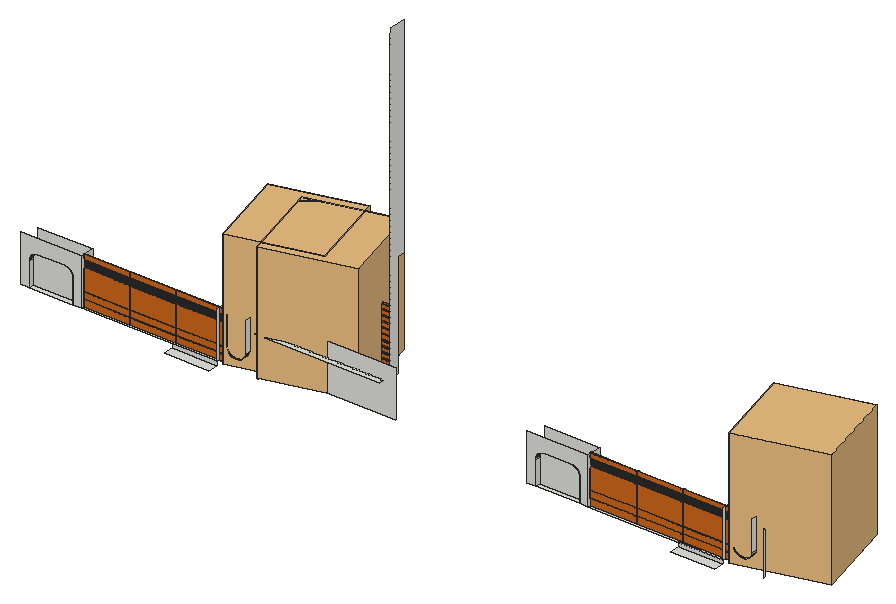
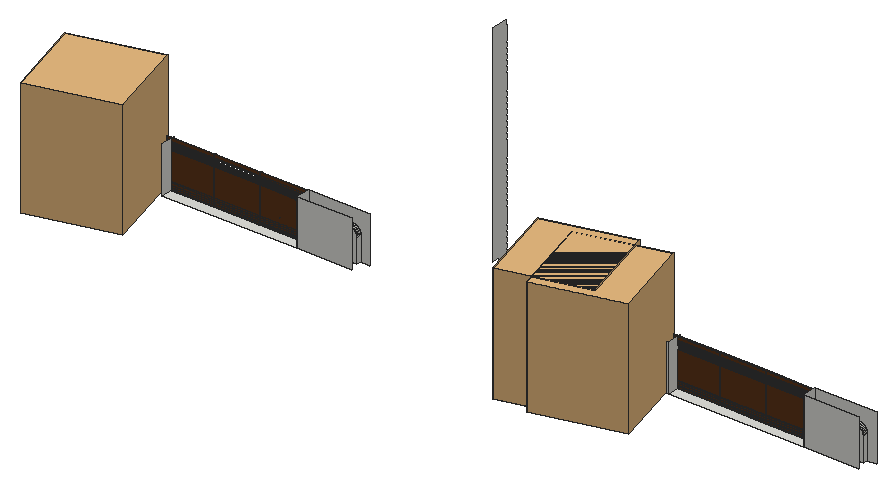
# SketchUp Ruby script. Lengths in inches.
U = 1.inch
M = Sketchup.active_model
def pt(a) = Geom::Point3d.new(a.map { |v| v * U })
def face(e, loops, mat)
  f = e.add_face(loops[0].map { |a| pt(a) })
  loops[1..].each { |l| e.add_face(l.map { |a| pt(a) }).erase! }
  f.material = f.back_material = mat if mat
  f
end
# faces: each face lists its corners as indices into pts; further lists are holes
def faces(e, pts, list, mat = nil) = list.each { |f| face(e, (f[0].is_a?(Array) ? f : [f]).map { |l| l.map { |i| pts[i] } }, mat) }
# xy, xz, yz: faces in a plane at the given z, y or x. An outline is a flat list of corners, or four numbers for a rectangle; further outlines are holes
def ring(l) = l.size == 4 ? [[l[0], l[1]], [l[2], l[1]], [l[2], l[3]], [l[0], l[3]]] : l.each_slice(2).to_a
def flat(e, list, mat, &to3) = list.each { |f| face(e, (f[0].is_a?(Array) ? f : [f]).map { |l| ring(l).map { |u, v| to3.(u, v) } }, mat) }
def xy(e, z, list, mat = nil) = flat(e, list, mat) { |x, y| [x, y, z] }
def xz(e, y, list, mat = nil) = flat(e, list, mat) { |x, z| [x, y, z] }
def yz(e, x, list, mat = nil) = flat(e, list, mat) { |y, z| [x, y, z] }
def lines(e, pts, list) = list.each { |a, b| e.add_line(pt(pts[a]), pt(pts[b])) }
# prism: a flat outline (further loops are holes) pulled along v
def prism(e, loops, v, mat = nil)
  f = face(e, loops, mat); d = Geom::Vector3d.new(v.map { |x| x * U })
  f.pushpull(f.normal.samedirection?(d) ? d.length : -d.length)
end
def box(e, o, s, mat = nil) = prism(e, [[o, [o[0] + s[0], o[1], o[2]], [o[0] + s[0], o[1] + s[1], o[2]], [o[0], o[1] + s[1], o[2]]]], [0, 0, s[2]], mat)
def at(x, y, z, deg = 0) = Geom::Transformation.translation(pt([x, y, z])) * Geom::Transformation.rotation(ORIGIN, Z_AXIS, deg.degrees)
def axes(o, x, y, z) = Geom::Transformation.new([*x, 0, *y, 0, *z, 0, *pt(o).to_a, 1])
def part(name) = M.definitions.add(name)
# library, detail: a bought-in or finely detailed component or shape, given as its bounding box
def library(name, o, s) = part(name).tap { |d| box(d.entities, o, s) }
def detail(e, o, s) = box(e.add_group.entities, o, s)
def put(e, d, t, mat = nil) = e.add_instance(d, t).tap { |i| i.material = mat if mat }
def group(e, t, mat = nil) = e.add_group.tap { |g| g.transformation = t; g.material = mat if mat }.entities
root = M.entities
M.materials.add("[0041_Chocolate]").color = [210, 105, 30]
M.materials.add("[Color M06]").color = [84, 84, 84]
M.materials.add("[Wood Veneer 01]2").color = [94, 55, 29]
c1 = part("Slatted screen panel")
xy(c1.entities,0,[[0,0,255.91,1.97]],"[Wood Veneer 01]2")
xy(c1.entities,16.54,[[0,1.18,255.91,1.97]],"[Wood Veneer 01]2")
xy(c1.entities,16.93,[[0,0,255.91,1.18]],"[Wood Veneer 01]2")
xy(c1.entities,17.78,[[0,0,255.91,1.18]],"[Wood Veneer 01]2")
xy(c1.entities,34.45,[[0,0,255.91,1.18]],"[Wood Veneer 01]2")
xy(c1.entities,35.07,[[0,0,255.91,1.18]],"[Wood Veneer 01]2")
xy(c1.entities,89.37,[[0,0,255.91,1.97]],"[Wood Veneer 01]2")
xy(c1.entities,92.91,[[0,0,255.91,1.97]],"[Wood Veneer 01]2")
xy(c1.entities,94.49,[[0,0,255.91,1.97]],"[Wood Veneer 01]2")
xy(c1.entities,97.64,[[0,0,255.91,1.97]],"[Wood Veneer 01]2")
xy(c1.entities,99.21,[[0,0,255.91,1.97]],"[Wood Veneer 01]2")
xy(c1.entities,102.36,[[0,0,255.91,1.97]],"[Wood Veneer 01]2")
xy(c1.entities,103.9375,[[0,0,255.91,1.97]],"[Wood Veneer 01]2")
xy(c1.entities,107.48,[[0,0,255.91,1.97]],"[Wood Veneer 01]2")
xy(c1.entities,119.29,[[0,0,255.91,1.97]],"[Wood Veneer 01]2")
xz(c1.entities,0,[[0,0,255.91,16.93],[0,17.78,255.91,34.45],[0,35.07,255.91,89.37],[0,92.91,255.91,94.49],[0,97.64,255.91,99.21],
  [0,102.36,255.91,103.9375],[0,107.48,255.91,119.29]],"[0041_Chocolate]")
xz(c1.entities,1.18,[[0,16.54,255.91,16.93],[0,16.93,255.91,17.78],[0,34.45,255.91,35.07]],"[Wood Veneer 01]2")
xz(c1.entities,1.97,[[0,0,255.91,1.57],[0,1.57,255.91,5.51],[0,5.51,255.91,7.09],[0,7.09,255.91,11.8125],[0,11.8125,255.91,16.54],
  [0,16.54,255.91,19.69],[0,19.69,255.91,89.37],[0,92.91,255.91,94.49],[0,97.64,255.91,99.21],[0,102.36,255.91,103.9375],
  [0,107.48,255.91,109.84],[0,109.84,255.91,119.29]],"[Wood Veneer 01]2")
yz(c1.entities,0,[[0,0,1.97,1.57],[0,1.57,1.97,5.51],[0,5.51,1.97,7.09],[0,7.09,1.97,11.8125],[0,11.8125,0,16.93,1.18,16.93,1.18,16.54,1.97,16.54,1.97,11.8125],
  [1.18,16.54,1.97,19.69],[0,17.78,0,34.45,1.18,34.45,1.18,35.07,0,35.07,0,89.37,1.97,89.37,1.97,19.69,1.18,19.69,1.18,17.78],[0,92.91,1.97,94.49],[0,97.64,1.97,99.21],[0,102.36,1.97,103.9375],
  [0,107.48,1.97,109.84],[0,109.84,1.97,119.29]],"[Wood Veneer 01]2")
yz(c1.entities,255.91,[[0,0,1.97,1.57],[0,1.57,1.97,5.51],[0,5.51,1.97,7.09],[0,7.09,1.97,11.8125],[0,11.8125,1.97,11.8125,1.97,16.54,1.18,16.54,1.18,16.93,0,16.93],
  [1.18,16.54,1.97,19.69],[0,17.78,1.18,17.78,1.18,19.69,1.97,19.69,1.97,89.37,0,89.37,0,35.07,1.18,35.07,1.18,34.45,0,34.45],[0,92.91,1.97,94.49],[0,97.64,1.97,99.21],[0,102.36,1.97,103.9375],
  [0,107.48,1.97,109.84],[0,109.84,1.97,119.29]],"[Wood Veneer 01]2")
p = [[255.91,1.97,103.9375],[255.91,1.97,107.48],[0,1.97,107.48],[0,1.97,103.9375],[0,1.97,92.91],[0,1.97,89.37],
  [255.91,1.97,99.21],[255.91,1.97,102.36],[255.91,1.97,89.37],[255.91,1.97,92.91],[0,1.97,97.64],[0,1.97,94.49],
  [0,1.97,102.36],[0,1.97,99.21],[255.91,1.97,94.49],[255.91,1.97,97.64],[240.94,0,5.51],[240.94,1.97,5.51]]
lines(c1.entities,p,[[0,1],[2,3],[4,5],[6,7],[8,9],[10,11],[12,13],[14,15],[16,17]])
c2 = library("Palm tree",[-4.09,-4.52,0],[193.52,193.51,258.93])
c3 = part("Palm+Tree")
put(c3.entities,c2,at(25.51,-21.81,0,15))
xy(root,0.73,[[705.71,876.83,762.73,889.52],[1361.21,876.83,1418.23,889.52]])
xy(root,6.125,[[520.36,889.52,577.24,895.77],[588.18,889.52,762.97,908.02],[1175.86,889.52,1232.74,895.77],[1243.68,889.52,1418.47,908.02],[916.04,971.36,921.96,983.34]])
xy(root,11.08,[[820.52,971.36,921.96,972.36]],"[0041_Chocolate]")
xy(root,13.1875,[[820.52,971.36,921.96,972.36]],"[0041_Chocolate]")
xy(root,18.14,[[820.52,971.36,921.96,972.36]],"[0041_Chocolate]")
xy(root,20.25,[[820.52,971.36,921.96,972.36]],"[0041_Chocolate]")
xy(root,25.2,[[820.52,971.36,921.96,972.36]],"[0041_Chocolate]")
xy(root,27.3125,[[820.52,971.36,921.96,972.36]],"[0041_Chocolate]")
xy(root,32.27,[[820.52,971.36,921.96,972.36]],"[0041_Chocolate]")
xy(root,34.375,[[820.52,971.36,921.96,972.36]],"[0041_Chocolate]")
xy(root,39.33,[[820.52,971.36,921.96,972.36]],"[0041_Chocolate]")
xy(root,41.4375,[[820.52,971.36,921.96,972.36]],"[0041_Chocolate]")
xy(root,46.39,[[820.52,971.36,921.96,972.36]],"[0041_Chocolate]")
xy(root,48,[[531.29,889.52,565.74,895.77],[1186.79,889.52,1221.24,895.77]])
xy(root,48.5,[[820.52,971.36,921.96,972.36]],"[0041_Chocolate]")
xy(root,53.45,[[820.52,971.36,921.96,972.36]],"[0041_Chocolate]")
xy(root,55.1875,[[811.8125,889.52,811.8125,894.77,813.4375,894.77,813.4375,895.77,814.1875,895.77,814.1875,894.77,817.4375,894.77,817.4375,895.77,818.1875,895.77,818.1875,894.77,821.4375,894.77,821.4375,895.77,822.1875,895.77,822.1875,894.77,825.4375,894.77,825.4375,895.77,826.1875,895.77,826.1875,894.77,829.4375,894.77,829.4375,895.77,830.1875,895.77,830.1875,894.77,833.4375,894.77,833.4375,895.77,834.1875,895.77,834.1875,894.77,837.4375,894.77,837.4375,895.77,838.1875,895.77,838.1875,894.77,841.4375,894.77,841.4375,895.77,842.1875,895.77,842.1875,894.77,845.4375,894.77,845.4375,895.77,846.1875,895.77,846.1875,894.77,849.4375,894.77,849.4375,895.77,850.1875,895.77,850.1875,894.77,853.4375,894.77,853.4375,895.77,854.1875,895.77,854.1875,894.77,857.4375,894.77,857.4375,895.77,858.1875,895.77,858.1875,894.77,861.4375,894.77,861.4375,895.77,862.1875,895.77,862.1875,894.77,865.4375,894.77,865.4375,895.77,866.1875,895.77,866.1875,894.77,869.4375,894.77,869.4375,895.77,870.1875,895.77,870.1875,894.77,873.4375,894.77,873.4375,895.77,874.1875,895.77,874.1875,894.77,877.4375,894.77,877.4375,895.77,878.1875,895.77,878.1875,894.77,881.4375,894.77,881.4375,895.77,882.1875,895.77,882.1875,894.77,885.4375,894.77,885.4375,895.77,886.1875,895.77,886.1875,894.77,889.4375,894.77,889.4375,895.77,890.1875,895.77,890.1875,894.77,893.4375,894.77,893.4375,895.77,894.1875,895.77,894.1875,894.77,897.4375,894.77,897.4375,895.77,898.1875,895.77,898.1875,894.77,901.4375,894.77,901.4375,895.77,902.1875,895.77,902.1875,894.77,905.4375,894.77,905.4375,895.77,906.1875,895.77,906.1875,894.77,909.4375,894.77,909.4375,895.77,910.1875,895.77,910.1875,894.77,913.4375,894.77,913.4375,895.77,914.1875,895.77,914.1875,894.77,917.4375,894.77,917.4375,895.77,918.1875,895.77,918.1875,894.77,921.4375,894.77,921.4375,895.77,922.1875,895.77,922.1875,894.77,925.4375,894.77,925.4375,895.77,926.1875,895.77,926.1875,894.77,929.4375,894.77,929.4375,895.77,930.1875,895.77,930.1875,894.77,933.4375,894.77,933.4375,895.77,934.1875,895.77,934.1875,894.77,937.4375,894.77,937.4375,895.77,938.1875,895.77,938.1875,894.77,941.4375,894.77,941.4375,895.77,942.1875,895.77,942.1875,894.77,945.4375,894.77,945.4375,895.77,946.1875,895.77,946.1875,894.77,949.4375,894.77,949.4375,895.77,950.1875,895.77,950.1875,894.77,953.4375,894.77,953.4375,895.77,954.1875,895.77,954.1875,894.77,957.4375,894.77,957.4375,895.77,958.1875,895.77,958.1875,894.77,961.4375,894.77,961.4375,895.77,962.1875,895.77,962.1875,894.77,965.4375,894.77,965.4375,895.77,966.1875,895.77,966.1875,894.77,969.4375,894.77,969.4375,895.77,970.1875,895.77,970.1875,894.77,973.4375,894.77,973.4375,889.52]])
xy(root,55.5625,[[820.52,971.36,921.96,972.36]],"[0041_Chocolate]")
xy(root,60.52,[[820.52,971.36,921.96,972.36]],"[0041_Chocolate]")
xy(root,62.625,[[820.52,971.36,921.96,972.36]],"[0041_Chocolate]")
xy(root,67.58,[[820.52,971.36,921.96,972.36]],"[0041_Chocolate]")
xy(root,69.6875,[[820.52,971.36,921.96,972.36]],"[0041_Chocolate]")
xy(root,74.64,[[820.52,971.36,856.72,972.36],[874.67,971.36,921.96,972.36]],"[0041_Chocolate]")
xy(root,76.75,[[820.52,971.36,851.63,972.36],[879.76,971.36,921.96,972.36]],"[0041_Chocolate]")
xy(root,81.7,[[820.52,971.36,844.79,972.36],[886.6,971.36,921.96,972.36]],"[0041_Chocolate]")
xy(root,83.8125,[[820.52,971.36,843.11,972.36],[888.28,971.36,921.96,972.36]],"[0041_Chocolate]")
xy(root,88.77,[[820.52,971.36,839.58,972.36],[891.8125,971.36,921.96,972.36]],"[0041_Chocolate]")
xz(root,889.52,[[705.71,0.73,762.73,6.125],[1361.21,0.73,1418.23,6.125],[508.71,6.125,520.36,6.125,520.36,37.07,520.45,38.5,520.73,39.9,521.19,41.25,521.82,42.53,522.62,43.72,523.5625,44.8,524.64,45.74,525.83,46.54,527.11,47.17,528.46,47.63,529.86,47.91,531.29,48,565.74,48,567.24,47.9,568.72,47.61,570.14,47.125,571.49,46.46,572.74,45.625,573.87,44.63,574.86,43.5,575.7,42.25,576.36,40.9,576.84,39.48,577.14,38.01,577.24,36.51,577.24,6.125,588.18,6.125,588.18,66.125,508.71,66.125],[1164.21,6.125,1175.86,6.125,1175.86,37.07,1175.95,38.5,1176.23,39.9,1176.69,41.25,1177.32,42.53,1178.12,43.72,1179.0625,44.8,1180.14,45.74,1181.33,46.54,1182.61,47.17,1183.96,47.63,1185.36,47.91,1186.79,48,1221.24,48,1222.74,47.9,1224.22,47.61,1225.64,47.125,1226.99,46.46,1228.24,45.625,1229.37,44.63,1230.36,43.5,1231.2,42.25,1231.86,40.9,1232.34,39.48,1232.64,38.01,1232.74,36.51,1232.74,6.125,1243.68,6.125,1243.68,66.125,1164.21,66.125]])
xz(root,895.77,[[810.1875,0,811.8125,55.1875],[1465.6875,0,1467.3125,55.1875],[520.36,6.125,577.24,6.125,577.24,36.51,577.14,38.01,576.84,39.48,576.36,40.9,575.7,42.25,574.86,43.5,573.87,44.63,572.74,45.625,571.49,46.46,570.14,47.125,568.72,47.61,567.24,47.9,565.74,48,531.29,48,529.86,47.91,528.46,47.63,527.11,47.17,525.83,46.54,524.64,45.74,523.5625,44.8,522.62,43.72,521.82,42.53,521.19,41.25,520.73,39.9,520.45,38.5,520.36,37.07],[1175.86,6.125,1232.74,6.125,1232.74,36.51,1232.64,38.01,1232.34,39.48,1231.86,40.9,1231.2,42.25,1230.36,43.5,1229.37,44.63,1228.24,45.625,1226.99,46.46,1225.64,47.125,1224.22,47.61,1222.74,47.9,1221.24,48,1186.79,48,1185.36,47.91,1183.96,47.63,1182.61,47.17,1181.33,46.54,1180.14,45.74,1179.0625,44.8,1178.12,43.72,1177.32,42.53,1176.69,41.25,1176.23,39.9,1175.95,38.5,1175.86,37.07]])
xz(root,895.77,[[788.25,16.91,791.05,17.23,793.71,18.17,796.09,19.69,798.06,21.71,799.52,24.11,800.41,26.79,800.41,66.125,776.1,66.125,776.1,26.79,776.98,24.11,778.45,21.71,780.42,19.69,782.8,18.17,785.45,17.23],[1443.75,16.91,1446.55,17.23,1449.21,18.17,1451.59,19.69,1453.56,21.71,1455.02,24.11,1455.91,26.79,1455.91,66.125,1431.6,66.125,1431.6,26.79,1432.48,24.11,1433.95,21.71,1435.92,19.69,1438.3,18.17,1440.95,17.23]],"[0041_Chocolate]")
xz(root,908.02,[[516.89,6.125,588.18,66.125],[762.97,6.125,979.81,66.125],[1172.39,6.125,1243.68,66.125]])
xz(root,971.36,[[820.52,6.125,921.96,11.08],[820.52,13.1875,921.96,18.14],[820.52,20.25,921.96,25.2],[820.52,27.3125,921.96,32.27],[820.52,34.375,921.96,39.33],
  [820.52,41.4375,921.96,46.39],[820.52,48.5,921.96,53.45],[820.52,55.5625,921.96,60.52],[820.52,62.625,921.96,67.58],[820.52,69.6875,921.96,69.6875,921.96,74.64,874.67,74.64,873.41,74.12,865.7,73.1,857.99,74.12,856.72,74.64,820.52,74.64],
  [820.52,76.75,851.63,76.75,850.8,77.09,844.79,81.7,820.52,81.7],[879.76,76.75,921.96,76.75,921.96,81.7,886.6,81.7,880.59,77.09],[820.52,83.8125,843.11,83.8125,839.9,88,839.58,88.77,820.52,88.77],[888.28,83.8125,921.96,83.8125,921.96,88.77,891.8125,88.77,891.49,88]],"[0041_Chocolate]")
xz(root,972.36,[[820.52,11.08,921.96,13.1875],[820.52,18.14,921.96,20.25],[820.52,25.2,921.96,27.3125],[820.52,32.27,921.96,34.375],[820.52,39.33,921.96,41.4375],
  [820.52,46.39,921.96,48.5],[820.52,53.45,921.96,55.5625],[820.52,60.52,921.96,62.625],[820.52,67.58,921.96,69.6875],[820.52,74.64,856.72,74.64,851.63,76.75,820.52,76.75],
  [874.67,74.64,921.96,74.64,921.96,76.75,879.76,76.75],[820.52,81.7,844.79,81.7,844.63,81.83,843.11,83.8125,820.52,83.8125],[886.6,81.7,921.96,81.7,921.96,83.8125,888.28,83.8125,886.76,81.83],[820.52,88.77,839.58,88.77,838.71,90.875,820.52,90.875],[891.8125,88.77,921.96,88.77,921.96,90.875,892.69,90.875]],"[0041_Chocolate]")
yz(root,520.36,[[889.52,6.125,895.77,37.07]])
yz(root,577.24,[[889.52,6.125,895.77,36.51]])
yz(root,588.18,[[889.52,6.125,908.02,66.125]])
yz(root,762.97,[[889.52,6.125,908.02,66.125]])
yz(root,776.1,[[889.52,26.79,895.77,66.125]])
yz(root,800.41,[[889.52,26.79,895.77,66.125]])
yz(root,811.8125,[[894.77,0,895.77,55.1875]])
yz(root,820.52,[[971.36,6.125,971.36,11.08,972.36,11.08,972.36,13.1875,971.36,13.1875,971.36,18.14,972.36,18.14,972.36,20.25,971.36,20.25,971.36,25.2,972.36,25.2,972.36,27.3125,971.36,27.3125,971.36,32.27,972.36,32.27,972.36,34.375,971.36,34.375,971.36,39.33,972.36,39.33,972.36,41.4375,971.36,41.4375,971.36,46.39,972.36,46.39,972.36,48.5,971.36,48.5,971.36,53.45,972.36,53.45,972.36,55.5625,971.36,55.5625,971.36,60.52,972.36,60.52,972.36,62.625,971.36,62.625,971.36,67.58,972.36,67.58,972.36,69.6875,971.36,69.6875,971.36,74.64,972.36,74.64,972.36,76.75,971.36,76.75,971.36,81.7,972.36,81.7,972.36,83.8125,971.36,83.8125,971.36,88.77,972.36,88.77,972.36,90.875,971.36,90.875,971.36,95.83,972.36,95.83,972.36,97.9375,971.36,97.9375,971.36,102.89,972.36,102.89,972.36,105,971.36,105,971.36,109.95,972.36,109.95,972.36,112.0625,971.36,112.0625,971.36,117.02,972.36,117.02,972.36,119.125,971.36,119.125,971.36,124.08,972.36,124.08,972.36,126.1875,971.36,126.1875,971.36,131.14,972.36,131.14,972.36,133.25,971.36,133.25,971.36,138.2,972.36,138.2,972.36,140.3125,971.36,140.3125,971.36,141.26,983.34,141.26,983.34,126.125,993.35,126.125,993.35,6.125]])
yz(root,921.96,[[971.36,6.125,983.34,6.125,983.34,141.26,993.35,141.26,993.35,411.82,972.36,411.82,972.36,405.64,971.36,405.64,971.36,400.6875,972.36,400.6875,972.36,398.77,971.36,398.77,971.36,393.8125,972.36,393.8125,972.36,391.89,971.36,391.89,971.36,386.9375,972.36,386.9375,972.36,385.02,971.36,385.02,971.36,380.0625,972.36,380.0625,972.36,378.14,971.36,378.14,971.36,373.1875,972.36,373.1875,972.36,371.27,971.36,371.27,971.36,366.3125,972.36,366.3125,972.36,364.2,971.36,364.2,971.36,359.25,972.36,359.25,972.36,357.14,971.36,357.14,971.36,352.1875,972.36,352.1875,972.36,350.08,971.36,350.08,971.36,345.125,972.36,345.125,972.36,343.02,971.36,343.02,971.36,338.0625,972.36,338.0625,972.36,335.95,971.36,335.95,971.36,331,972.36,331,972.36,328.89,971.36,328.89,971.36,323.9375,972.36,323.9375,972.36,321.83,971.36,321.83,971.36,316.875,972.36,316.875,972.36,314.77,971.36,314.77,971.36,309.8125,972.36,309.8125,972.36,307.7,971.36,307.7,971.36,302.75,972.36,302.75,972.36,300.64,971.36,300.64,971.36,295.6875,972.36,295.6875,972.36,293.58,971.36,293.58,971.36,288.625,972.36,288.625,972.36,286.52,971.36,286.52,971.36,281.5625,972.36,281.5625,972.36,279.45,971.36,279.45,971.36,274.5,972.36,274.5,972.36,272.39,971.36,272.39,971.36,267.4375,972.36,267.4375,972.36,265.33,971.36,265.33,971.36,260.375,972.36,260.375,972.36,258.27,971.36,258.27,971.36,253.3125,972.36,253.3125,972.36,251.2,971.36,251.2,971.36,246.25,972.36,246.25,972.36,244.14,971.36,244.14,971.36,239.1875,972.36,239.1875,972.36,237.08,971.36,237.08,971.36,232.125,972.36,232.125,972.36,230.02,971.36,230.02,971.36,225.0625,972.36,225.0625,972.36,222.95,971.36,222.95,971.36,218,972.36,218,972.36,215.89,971.36,215.89,971.36,210.9375,972.36,210.9375,972.36,208.83,971.36,208.83,971.36,203.875,972.36,203.875,972.36,201.77,971.36,201.77,971.36,196.8125,972.36,196.8125,972.36,194.7,971.36,194.7,971.36,189.75,972.36,189.75,972.36,187.64,971.36,187.64,971.36,182.6875,972.36,182.6875,972.36,180.58,971.36,180.58,971.36,175.625,972.36,175.625,972.36,173.52,971.36,173.52,971.36,168.5625,972.36,168.5625,972.36,166.45,971.36,166.45,971.36,161.5,972.36,161.5,972.36,159.39,971.36,159.39,971.36,154.4375,972.36,154.4375,972.36,152.33,971.36,152.33,971.36,147.375,972.36,147.375,972.36,145.27,971.36,145.27,971.36,140.3125,972.36,140.3125,972.36,138.2,971.36,138.2,971.36,133.25,972.36,133.25,972.36,131.14,971.36,131.14,971.36,126.1875,972.36,126.1875,972.36,124.08,971.36,124.08,971.36,119.125,972.36,119.125,972.36,117.02,971.36,117.02,971.36,112.0625,972.36,112.0625,972.36,109.95,971.36,109.95,971.36,105,972.36,105,972.36,102.89,971.36,102.89,971.36,97.9375,972.36,97.9375,972.36,95.83,971.36,95.83,971.36,90.875,972.36,90.875,972.36,88.77,971.36,88.77,971.36,83.8125,972.36,83.8125,972.36,81.7,971.36,81.7,971.36,76.75,972.36,76.75,972.36,74.64,971.36,74.64,971.36,69.6875,972.36,69.6875,972.36,67.58,971.36,67.58,971.36,62.625,972.36,62.625,972.36,60.52,971.36,60.52,971.36,55.5625,972.36,55.5625,972.36,53.45,971.36,53.45,971.36,48.5,972.36,48.5,972.36,46.39,971.36,46.39,971.36,41.4375,972.36,41.4375,972.36,39.33,971.36,39.33,971.36,34.375,972.36,34.375,972.36,32.27,971.36,32.27,971.36,27.3125,972.36,27.3125,972.36,25.2,971.36,25.2,971.36,20.25,972.36,20.25,972.36,18.14,971.36,18.14,971.36,13.1875,972.36,13.1875,972.36,11.08,971.36,11.08]])
yz(root,1175.86,[[889.52,6.125,895.77,37.07]])
yz(root,1232.74,[[889.52,6.125,895.77,36.51]])
yz(root,1243.68,[[889.52,6.125,908.02,66.125]])
yz(root,1418.47,[[889.52,6.125,908.02,66.125]])
yz(root,1431.6,[[889.52,26.79,895.77,66.125]])
yz(root,1455.91,[[889.52,26.79,895.77,66.125]])
yz(root,1467.3125,[[894.77,0,895.77,55.1875]])
p = [[788.25,895.77,16.91],[785.45,895.77,17.23],[785.45,889.52,17.23],[788.25,889.52,16.91],[791.05,895.77,17.23],[791.05,889.52,17.23],
  [1443.75,895.77,16.91],[1440.95,895.77,17.23],[1440.95,889.52,17.23],[1443.75,889.52,16.91],[1446.55,895.77,17.23],[1446.55,889.52,17.23],
  [782.8,895.77,18.17],[782.8,889.52,18.17],[793.71,895.77,18.17],[793.71,889.52,18.17],[1438.3,895.77,18.17],[1438.3,889.52,18.17],
  [1449.21,895.77,18.17],[1449.21,889.52,18.17],[780.42,895.77,19.69],[780.42,889.52,19.69],[796.09,895.77,19.69],[796.09,889.52,19.69],
  [1435.92,895.77,19.69],[1435.92,889.52,19.69],[1451.59,895.77,19.69],[1451.59,889.52,19.69],[778.45,895.77,21.71],[778.45,889.52,21.71],
  [798.06,895.77,21.71],[798.06,889.52,21.71],[1433.95,895.77,21.71],[1433.95,889.52,21.71],[1453.56,895.77,21.71],[1453.56,889.52,21.71],
  [776.98,895.77,24.11],[776.98,889.52,24.11],[799.52,895.77,24.11],[799.52,889.52,24.11],[1432.48,895.77,24.11],[1432.48,889.52,24.11],
  [1455.02,895.77,24.11],[1455.02,889.52,24.11],[776.1,895.77,26.79],[776.1,889.52,26.79],[800.41,895.77,26.79],[800.41,889.52,26.79],
  [1431.6,895.77,26.79],[1431.6,889.52,26.79],[1455.91,895.77,26.79],[1455.91,889.52,26.79],[577.14,895.77,38.01],[577.24,895.77,36.51],
  [577.24,889.52,36.51],[577.14,889.52,38.01],[1232.64,895.77,38.01],[1232.74,895.77,36.51],[1232.74,889.52,36.51],[1232.64,889.52,38.01],
  [520.36,895.77,37.07],[520.45,895.77,38.5],[520.45,889.52,38.5],[520.36,889.52,37.07],[1175.86,895.77,37.07],[1175.95,895.77,38.5],
  [1175.95,889.52,38.5],[1175.86,889.52,37.07],[576.84,895.77,39.48],[576.84,889.52,39.48],[1232.34,895.77,39.48],[1232.34,889.52,39.48],
  [520.73,895.77,39.9],[520.73,889.52,39.9],[1176.23,895.77,39.9],[1176.23,889.52,39.9],[576.36,895.77,40.9],[576.36,889.52,40.9],
  [1231.86,895.77,40.9],[1231.86,889.52,40.9],[521.19,895.77,41.25],[521.19,889.52,41.25],[1176.69,895.77,41.25],[1176.69,889.52,41.25],
  [575.7,895.77,42.25],[575.7,889.52,42.25],[1231.2,895.77,42.25],[1231.2,889.52,42.25],[521.82,895.77,42.53],[521.82,889.52,42.53],
  [1177.32,895.77,42.53],[1177.32,889.52,42.53],[574.86,895.77,43.5],[574.86,889.52,43.5],[1230.36,895.77,43.5],[1230.36,889.52,43.5],
  [522.62,895.77,43.72],[522.62,889.52,43.72],[1178.12,895.77,43.72],[1178.12,889.52,43.72],[573.87,895.77,44.63],[573.87,889.52,44.63],
  [1229.37,895.77,44.63],[1229.37,889.52,44.63],[523.5625,895.77,44.8],[523.5625,889.52,44.8],[1179.0625,895.77,44.8],[1179.0625,889.52,44.8],
  [572.74,895.77,45.625],[572.74,889.52,45.625],[1228.24,895.77,45.625],[1228.24,889.52,45.625],[524.64,895.77,45.74],[524.64,889.52,45.74],
  [1180.14,895.77,45.74],[1180.14,889.52,45.74],[571.49,895.77,46.46],[571.49,889.52,46.46],[1226.99,895.77,46.46],[1226.99,889.52,46.46],
  [525.83,895.77,46.54],[525.83,889.52,46.54],[1181.33,895.77,46.54],[1181.33,889.52,46.54],[527.11,895.77,47.17],[527.11,889.52,47.17],
  [570.14,895.77,47.125],[570.14,889.52,47.125],[1182.61,895.77,47.17],[1182.61,889.52,47.17],[1225.64,895.77,47.125],[1225.64,889.52,47.125],
  [568.72,895.77,47.61],[568.72,889.52,47.61],[1224.22,895.77,47.61],[1224.22,889.52,47.61],[528.46,895.77,47.63],[528.46,889.52,47.63],
  [1183.96,895.77,47.63],[1183.96,889.52,47.63],[529.86,895.77,47.91],[529.86,889.52,47.91],[567.24,895.77,47.9],[567.24,889.52,47.9],
  [1185.36,895.77,47.91],[1185.36,889.52,47.91],[1222.74,895.77,47.9],[1222.74,889.52,47.9],[531.29,895.77,48],[531.29,889.52,48],
  [565.74,895.77,48],[565.74,889.52,48],[1186.79,895.77,48],[1186.79,889.52,48],[1221.24,895.77,48],[1221.24,889.52,48],
  [844.79,986.55,81.7],[844.79,972.36,81.7],[844.79,971.36,81.7],[850.8,971.36,77.09],[850.8,986.55,77.09],[839.9,986.55,88],
  [839.9,971.36,88],[843.11,971.36,83.8125],[843.11,972.36,83.8125],[843.11,986.55,83.8125],[839.58,986.55,88.77],[839.58,972.36,88.77],
  [839.58,971.36,88.77]]
faces(root,p,[[0,1,2,3],[4,0,3,5],[6,7,8,9],[10,6,9,11],[1,12,13,2],[14,4,5,15],[7,16,17,8],[18,10,11,19],
  [12,20,21,13],[22,14,15,23],[16,24,25,17],[26,18,19,27],[20,28,29,21],[30,22,23,31],[24,32,33,25],[34,26,27,35],
  [28,36,37,29],[38,30,31,39],[32,40,41,33],[42,34,35,43],[36,44,45,37],[46,38,39,47],[40,48,49,41],[50,42,43,51],
  [52,53,54,55],[56,57,58,59],[60,61,62,63],[64,65,66,67],[68,52,55,69],[70,56,59,71],[61,72,73,62],[65,74,75,66],
  [76,68,69,77],[78,70,71,79],[72,80,81,73],[74,82,83,75],[84,76,77,85],[86,78,79,87],[80,88,89,81],[82,90,91,83],
  [92,84,85,93],[94,86,87,95],[88,96,97,89],[90,98,99,91],[100,92,93,101],[102,94,95,103],[96,104,105,97],[98,106,107,99],
  [108,100,101,109],[110,102,103,111],[104,112,113,105],[106,114,115,107],[116,108,109,117],[118,110,111,119],[112,120,121,113],[114,122,123,115],
  [120,124,125,121],[126,116,117,127],[122,128,129,123],[130,118,119,131],[132,126,127,133],[134,130,131,135],[124,136,137,125],[128,138,139,129],
  [136,140,141,137],[142,132,133,143],[138,144,145,139],[146,134,135,147],[140,148,149,141],[150,142,143,151],[144,152,153,145],[154,146,147,155]])
faces(root,p,[[156,157,158,159,160],[161,162,163,164,165],[166,167,168,162,161]],"[Color M06]")
put(root,c1,axes([588.27,892.77,6.125],[0.23355,0,0],[0,0.5124,0],[0,0,0.5124]),"[0041_Chocolate]")
put(root,c1,axes([648.04,892.77,6.125],[0.23355,0,0],[0,0.5124,0],[0,0,0.5124]),"[0041_Chocolate]")
put(root,c1,axes([707.81,892.77,6.125],[0.23355,0,0],[0,0.5124,0],[0,0,0.5124]),"[0041_Chocolate]")
put(root,c1,axes([1243.77,892.77,6.125],[0.23355,0,0],[0,0.5124,0],[0,0,0.5124]),"[0041_Chocolate]")
put(root,c1,axes([1303.54,892.77,6.125],[0.23355,0,0],[0,0.5124,0],[0,0,0.5124]),"[0041_Chocolate]")
put(root,c1,axes([1363.31,892.77,6.125],[0.23355,0,0],[0,0.5124,0],[0,0,0.5124]),"[0041_Chocolate]")
put(root,c3,axes([758.61,903.83,6.125],[0.58344,0,0],[0,0.58344,0],[0,0,0.58344]),"[Color M06]")
put(root,c3,axes([802.42,903.83,6.125],[0.58344,0,0],[0,0.58344,0],[0,0,0.58344]),"[Color M06]")
put(root,c3,axes([1414.11,903.83,6.125],[0.58344,0,0],[0,0.58344,0],[0,0,0.58344]),"[Color M06]")
